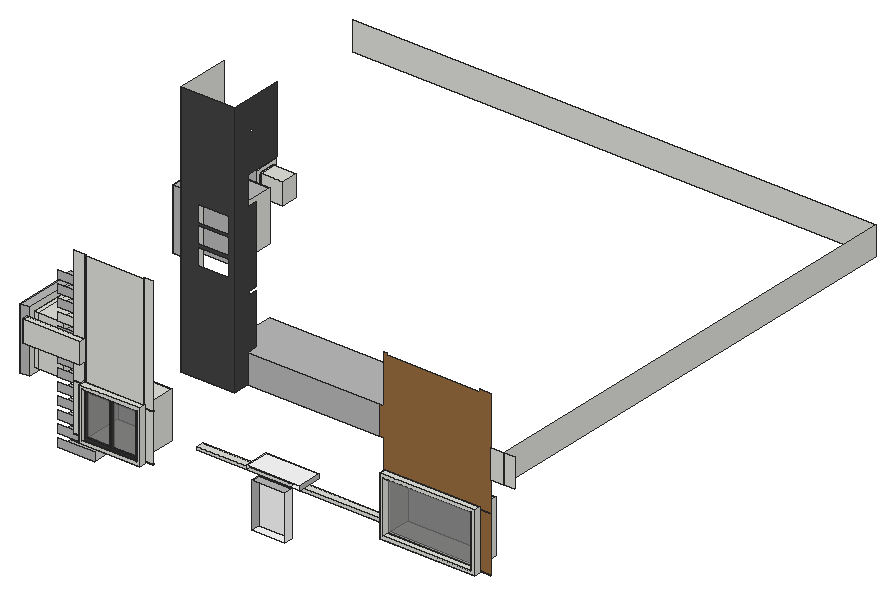
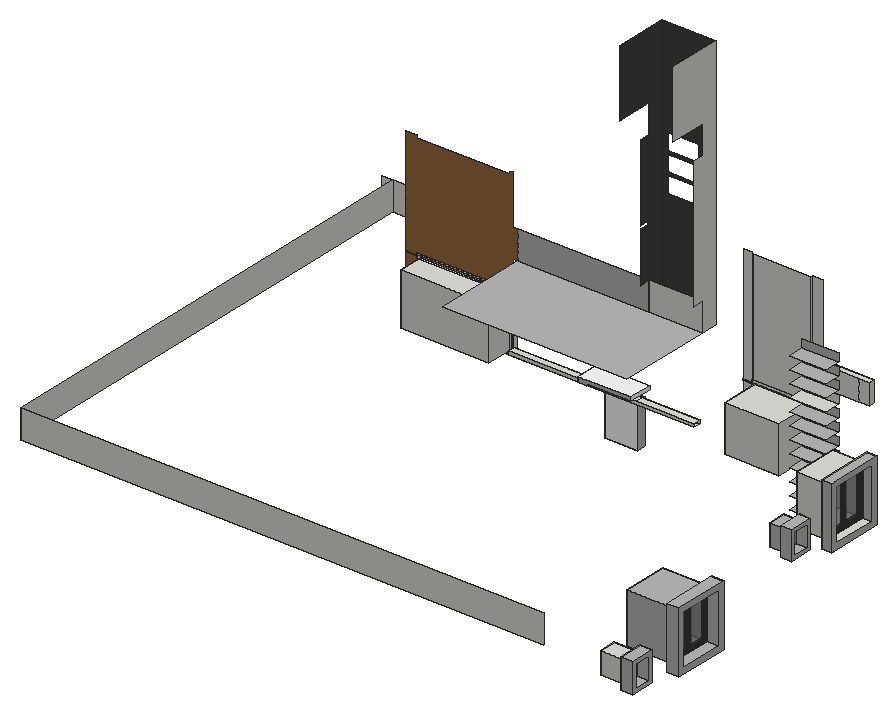
# SketchUp Ruby script. Lengths in inches.
U = 1.inch
M = Sketchup.active_model
def pt(a) = Geom::Point3d.new(a.map { |v| v * U })
def face(e, loops, mat)
  f = e.add_face(loops[0].map { |a| pt(a) })
  loops[1..].each { |l| e.add_face(l.map { |a| pt(a) }).erase! }
  f.material = f.back_material = mat if mat
  f
end
# faces: each face lists its corners as indices into pts; further lists are holes
def faces(e, pts, list, mat = nil) = list.each { |f| face(e, (f[0].is_a?(Array) ? f : [f]).map { |l| l.map { |i| pts[i] } }, mat) }
# xy, xz, yz: faces in a plane at the given z, y or x. An outline is a flat list of corners, or four numbers for a rectangle; further outlines are holes
def ring(l) = l.size == 4 ? [[l[0], l[1]], [l[2], l[1]], [l[2], l[3]], [l[0], l[3]]] : l.each_slice(2).to_a
def flat(e, list, mat, &to3) = list.each { |f| face(e, (f[0].is_a?(Array) ? f : [f]).map { |l| ring(l).map { |u, v| to3.(u, v) } }, mat) }
def xy(e, z, list, mat = nil) = flat(e, list, mat) { |x, y| [x, y, z] }
def xz(e, y, list, mat = nil) = flat(e, list, mat) { |x, z| [x, y, z] }
def yz(e, x, list, mat = nil) = flat(e, list, mat) { |y, z| [x, y, z] }
def lines(e, pts, list) = list.each { |a, b| e.add_line(pt(pts[a]), pt(pts[b])) }
# prism: a flat outline (further loops are holes) pulled along v
def prism(e, loops, v, mat = nil)
  f = face(e, loops, mat); d = Geom::Vector3d.new(v.map { |x| x * U })
  f.pushpull(f.normal.samedirection?(d) ? d.length : -d.length)
end
def box(e, o, s, mat = nil) = prism(e, [[o, [o[0] + s[0], o[1], o[2]], [o[0] + s[0], o[1] + s[1], o[2]], [o[0], o[1] + s[1], o[2]]]], [0, 0, s[2]], mat)
def at(x, y, z, deg = 0) = Geom::Transformation.translation(pt([x, y, z])) * Geom::Transformation.rotation(ORIGIN, Z_AXIS, deg.degrees)
def axes(o, x, y, z) = Geom::Transformation.new([*x, 0, *y, 0, *z, 0, *pt(o).to_a, 1])
def part(name) = M.definitions.add(name)
# library, detail: a bought-in or finely detailed component or shape, given as its bounding box
def library(name, o, s) = part(name).tap { |d| box(d.entities, o, s) }
def detail(e, o, s) = box(e.add_group.entities, o, s)
def put(e, d, t, mat = nil) = e.add_instance(d, t).tap { |i| i.material = mat if mat }
def group(e, t, mat = nil) = e.add_group.tap { |g| g.transformation = t; g.material = mat if mat }.entities
root = M.entities
M.materials.add("Generic").color = [155, 110, 63]
M.materials.add("Generic\#2").color = [186, 186, 186]
M.materials.add("[Color M00]").color = [255, 255, 255]
M.materials.add("[Color M07]").color = [58, 58, 58]
M.materials.add("[Granite Dark Gray]").color = [68, 67, 67]
M.materials.add("[Translucent Glass Gray]").color = [127, 127, 127]
M.materials["[Translucent Glass Gray]"].alpha = 0.58
M.materials.add("[Translucent Glass Gray]1").color = [127, 127, 127]
M.materials["[Translucent Glass Gray]1"].alpha = 0.5
c1 = part("Group\#1")
xy(c1.entities,0,[[0,0,46.77,20.375]])
xz(c1.entities,0,[[0,0,46.77,11.0625]])
c2 = part("Group\#3")
xy(c2.entities,0,[[0,0,70.4375,6]],"[Color M07]")
xy(c2.entities,2.83,[[2.83,0,33.8,3],[36.63,0,67.61,3]],"[Color M07]")
xy(c2.entities,56.73,[[2.83,0,33.8,3],[36.63,0,67.61,3]],"[Color M07]")
xy(c2.entities,59.5625,[[0,0,70.4375,6]],"[Color M07]")
xz(c2.entities,0,[[[0,0,70.4375,59.5625],[2.83,2.83,33.8,56.73],[36.63,2.83,67.61,56.73]]],"[Color M07]")
xz(c2.entities,3,[[2.83,2.83,33.8,56.73],[36.63,2.83,67.61,56.73]],"[Translucent Glass Gray]")
xz(c2.entities,6,[[0,0,70.4375,59.5625]],"[Translucent Glass Gray]")
yz(c2.entities,0,[[0,0,6,59.5625]],"[Color M07]")
yz(c2.entities,2.83,[[0,2.83,3,56.73]],"[Color M07]")
yz(c2.entities,33.8,[[0,2.83,3,56.73]],"[Color M07]")
yz(c2.entities,36.63,[[0,2.83,3,56.73]],"[Color M07]")
yz(c2.entities,67.61,[[0,2.83,3,56.73]],"[Color M07]")
yz(c2.entities,70.4375,[[0,0,6,59.5625]],"[Color M07]")
c3 = part("Group\#4")
xy(c3.entities,0,[[0,0,6,57.4375]],"[Color M07]")
xy(c3.entities,5.48,[[0,5.48,3,25.98],[0,31.46,3,51.96]],"[Color M07]")
xy(c3.entities,59.46,[[0,5.48,3,25.98],[0,31.46,3,51.96]],"[Color M07]")
xy(c3.entities,64.9375,[[0,0,6,57.4375]],"[Color M07]")
xz(c3.entities,0,[[0,0,6,64.9375]],"[Color M07]")
xz(c3.entities,5.48,[[0,5.48,3,59.46]],"[Color M07]")
xz(c3.entities,25.98,[[0,5.48,3,59.46]],"[Color M07]")
xz(c3.entities,31.46,[[0,5.48,3,59.46]],"[Color M07]")
xz(c3.entities,51.96,[[0,5.48,3,59.46]],"[Color M07]")
xz(c3.entities,57.4375,[[0,0,6,64.9375]],"[Color M07]")
yz(c3.entities,0,[[[0,0,57.4375,64.9375],[31.46,5.48,51.96,59.46],[5.48,5.48,25.98,59.46]]],"[Color M07]")
yz(c3.entities,3,[[5.48,5.48,25.98,59.46],[31.46,5.48,51.96,59.46]],"[Translucent Glass Gray]1")
yz(c3.entities,6,[[0,0,57.4375,64.9375]],"[Translucent Glass Gray]1")
c4 = part("Group\#2")
xy(c4.entities,0,[[0,0,113.875,3]])
xy(c4.entities,67.5625,[[0,0,113.875,3]])
xz(c4.entities,0,[[0,0,113.875,67.5625]],"[Translucent Glass Gray]")
xz(c4.entities,3,[[0,0,113.875,67.5625]],"[Translucent Glass Gray]")
yz(c4.entities,0,[[0,0,3,67.5625]])
yz(c4.entities,113.875,[[0,0,3,67.5625]])
c5 = part("Group\#5")
xy(c5.entities,0,[[0,0,3,21.5625]])
xy(c5.entities,28.3125,[[0,0,3,21.5625]])
xz(c5.entities,0,[[0,0,3,28.3125]])
xz(c5.entities,21.5625,[[0,0,3,28.3125]])
yz(c5.entities,0,[[0,0,21.5625,28.3125]],"[Translucent Glass Gray]1")
yz(c5.entities,3,[[0,0,21.5625,28.3125]],"[Translucent Glass Gray]1")
xy(root,621.53,[[370.16,118.5625,412.84,129.4375]],"[Color M00]")
xy(root,663.96,[[0,454.08,15.3125,525.8]],"Generic\#2")
xy(root,664.625,[[170.35,89.25,249.19,97.25],[171.66,97.25,172.16,98.375],[247.01,97.25,247.51,98.375]])
xy(root,666.77,[[36.4375,161.95,48.5,234.18]],"Generic\#2")
xy(root,667,[[157.47,97.25,170.35,98],[249.19,97.25,259.3125,98]])
xy(root,667.5,[[157.47,97.25,170.35,98],[249.19,97.25,259.3125,98]])
xy(root,668.33,[[174.55,89.25,244.99,97.25],[174.55,97.25,244.99,145.8125]])
xy(root,670.65,[[536.25,116.625,658.53,124.5]])
xy(root,671.1,[[0,461.22,72.5625,518.66]],"Generic\#2")
xy(root,674.16,[[36.4375,169.34,48.5,226.78],[48.5,169.34,87,226.78]])
xy(root,674.85,[[540.45,116.625,654.33,124.5],[540.45,124.5,654.33,156.8125]])
xy(root,675.92,[[0,569.11,15.3125,600.66]],"Generic\#2")
xy(root,678.86,[[370.16,118.5625,412.84,129.4375]],"Generic\#2")
xy(root,679.96,[[512.54,132.04,512.75,132.07,512.95,132.15,513.12,132.28,513.25,132.45,513.33,132.64,513.36,132.85,513.33,133.06,513.25,133.26,513.12,133.43,512.95,133.56,512.75,133.64,512.54,133.67,512.33,133.64,512.14,133.56,511.97,133.43,511.84,133.26,511.76,133.06,511.73,132.85,511.76,132.64,511.84,132.45,511.97,132.28,512.14,132.15,512.33,132.07],[518.54,132.04,518.75,132.07,518.95,132.15,519.12,132.28,519.25,132.45,519.33,132.64,519.36,132.85,519.33,133.06,519.25,133.26,519.12,133.43,518.95,133.56,518.75,133.64,518.54,133.67,518.33,133.64,518.14,133.56,517.97,133.43,517.84,133.26,517.76,133.06,517.73,132.85,517.76,132.64,517.84,132.45,517.97,132.28,518.14,132.15,518.33,132.07]])
xy(root,680.58,[[[290.4375,129.43,528.75,138.74],[506.67,132.04,506.88,132.07,507.07,132.15,507.24,132.28,507.37,132.45,507.45,132.64,507.48,132.85,507.45,133.06,507.37,133.26,507.24,133.43,507.07,133.56,506.88,133.64,506.67,133.67,506.46,133.64,506.26,133.56,506.09,133.43,505.96,133.26,505.88,133.06,505.86,132.85,505.88,132.64,505.96,132.45,506.09,132.28,506.26,132.15,506.46,132.07],[500.86,132.04,501.07,132.07,501.26,132.15,501.43,132.28,501.56,132.45,501.64,132.64,501.67,132.85,501.64,133.06,501.56,133.26,501.43,133.43,501.26,133.56,501.07,133.64,500.86,133.67,500.64,133.64,500.45,133.56,500.28,133.43,500.15,133.26,500.07,133.06,500.04,132.85,500.07,132.64,500.15,132.45,500.28,132.28,500.45,132.15,500.64,132.07],[494.92,132.04,495.13,132.07,495.32,132.15,495.49,132.28,495.62,132.45,495.7,132.64,495.73,132.85,495.7,133.06,495.62,133.26,495.49,133.43,495.32,133.56,495.13,133.64,494.92,133.67,494.71,133.64,494.51,133.56,494.34,133.43,494.21,133.26,494.13,133.06,494.11,132.85,494.13,132.64,494.21,132.45,494.34,132.28,494.51,132.15,494.71,132.07],[488.98,132.04,489.19,132.07,489.39,132.15,489.55,132.28,489.68,132.45,489.77,132.64,489.79,132.85,489.77,133.06,489.68,133.26,489.55,133.43,489.39,133.56,489.19,133.64,488.98,133.67,488.77,133.64,488.57,133.56,488.41,133.43,488.28,133.26,488.2,133.06,488.17,132.85,488.2,132.64,488.28,132.45,488.41,132.28,488.57,132.15,488.77,132.07],[483.11,132.04,483.32,132.07,483.51,132.15,483.68,132.28,483.81,132.45,483.89,132.64,483.92,132.85,483.89,133.06,483.81,133.26,483.68,133.43,483.51,133.56,483.32,133.64,483.11,133.67,482.89,133.64,482.7,133.56,482.53,133.43,482.4,133.26,482.32,133.06,482.29,132.85,482.32,132.64,482.4,132.45,482.53,132.28,482.7,132.15,482.89,132.07],[477.23,132.04,477.44,132.07,477.64,132.15,477.8,132.28,477.93,132.45,478.02,132.64,478.04,132.85,478.02,133.06,477.93,133.26,477.8,133.43,477.64,133.56,477.44,133.64,477.23,133.67,477.02,133.64,476.82,133.56,476.66,133.43,476.53,133.26,476.45,133.06,476.42,132.85,476.45,132.64,476.53,132.45,476.66,132.28,476.82,132.15,477.02,132.07],[471.54,132.04,471.75,132.07,471.95,132.15,472.12,132.28,472.25,132.45,472.33,132.64,472.36,132.85,472.33,133.06,472.25,133.26,472.12,133.43,471.95,133.56,471.75,133.64,471.54,133.67,471.33,133.64,471.14,133.56,470.97,133.43,470.84,133.26,470.76,133.06,470.73,132.85,470.76,132.64,470.84,132.45,470.97,132.28,471.14,132.15,471.33,132.07],[465.54,132.04,465.75,132.07,465.95,132.15,466.12,132.28,466.25,132.45,466.33,132.64,466.36,132.85,466.33,133.06,466.25,133.26,466.12,133.43,465.95,133.56,465.75,133.64,465.54,133.67,465.33,133.64,465.14,133.56,464.97,133.43,464.84,133.26,464.76,133.06,464.73,132.85,464.76,132.64,464.84,132.45,464.97,132.28,465.14,132.15,465.33,132.07],[459.48,132.04,459.69,132.07,459.89,132.15,460.05,132.28,460.18,132.45,460.27,132.64,460.29,132.85,460.27,133.06,460.18,133.26,460.05,133.43,459.89,133.56,459.69,133.64,459.48,133.67,459.27,133.64,459.07,133.56,458.91,133.43,458.78,133.26,458.7,133.06,458.67,132.85,458.7,132.64,458.78,132.45,458.91,132.28,459.07,132.15,459.27,132.07],[453.86,132.04,454.07,132.07,454.26,132.15,454.43,132.28,454.56,132.45,454.64,132.64,454.67,132.85,454.64,133.06,454.56,133.26,454.43,133.43,454.26,133.56,454.07,133.64,453.86,133.67,453.64,133.64,453.45,133.56,453.28,133.43,453.15,133.26,453.07,133.06,453.04,132.85,453.07,132.64,453.15,132.45,453.28,132.28,453.45,132.15,453.64,132.07],[447.98,132.04,448.19,132.07,448.39,132.15,448.55,132.28,448.68,132.45,448.77,132.64,448.79,132.85,448.77,133.06,448.68,133.26,448.55,133.43,448.39,133.56,448.19,133.64,447.98,133.67,447.77,133.64,447.57,133.56,447.41,133.43,447.28,133.26,447.2,133.06,447.17,132.85,447.2,132.64,447.28,132.45,447.41,132.28,447.57,132.15,447.77,132.07],[442.11,132.04,442.32,132.07,442.51,132.15,442.68,132.28,442.81,132.45,442.89,132.64,442.92,132.85,442.89,133.06,442.81,133.26,442.68,133.43,442.51,133.56,442.32,133.64,442.11,133.67,441.89,133.64,441.7,133.56,441.53,133.43,441.4,133.26,441.32,133.06,441.29,132.85,441.32,132.64,441.4,132.45,441.53,132.28,441.7,132.15,441.89,132.07],[436.11,132.04,436.32,132.07,436.51,132.15,436.68,132.28,436.81,132.45,436.89,132.64,436.92,132.85,436.89,133.06,436.81,133.26,436.68,133.43,436.51,133.56,436.32,133.64,436.11,133.67,435.89,133.64,435.7,133.56,435.53,133.43,435.4,133.26,435.32,133.06,435.29,132.85,435.32,132.64,435.4,132.45,435.53,132.28,435.7,132.15,435.89,132.07],[430.54,132.04,430.75,132.07,430.95,132.15,431.12,132.28,431.25,132.45,431.33,132.64,431.36,132.85,431.33,133.06,431.25,133.26,431.12,133.43,430.95,133.56,430.75,133.64,430.54,133.67,430.33,133.64,430.14,133.56,429.97,133.43,429.84,133.26,429.76,133.06,429.73,132.85,429.76,132.64,429.84,132.45,429.97,132.28,430.14,132.15,430.33,132.07],[424.36,132.04,424.57,132.07,424.76,132.15,424.93,132.28,425.06,132.45,425.14,132.64,425.17,132.85,425.14,133.06,425.06,133.26,424.93,133.43,424.76,133.56,424.57,133.64,424.36,133.67,424.14,133.64,423.95,133.56,423.78,133.43,423.65,133.26,423.57,133.06,423.54,132.85,423.57,132.64,423.65,132.45,423.78,132.28,423.95,132.15,424.14,132.07],[418.54,132.04,418.75,132.07,418.95,132.15,419.12,132.28,419.25,132.45,419.33,132.64,419.36,132.85,419.33,133.06,419.25,133.26,419.12,133.43,418.95,133.56,418.75,133.64,418.54,133.67,418.33,133.64,418.14,133.56,417.97,133.43,417.84,133.26,417.76,133.06,417.73,132.85,417.76,132.64,417.84,132.45,417.97,132.28,418.14,132.15,418.33,132.07],[412.67,132.04,412.88,132.07,413.07,132.15,413.24,132.28,413.37,132.45,413.45,132.64,413.48,132.85,413.45,133.06,413.37,133.26,413.24,133.43,413.07,133.56,412.88,133.64,412.67,133.67,412.46,133.64,412.26,133.56,412.09,133.43,411.96,133.26,411.88,133.06,411.86,132.85,411.88,132.64,411.96,132.45,412.09,132.28,412.26,132.15,412.46,132.07],[406.79,132.04,407,132.07,407.2,132.15,407.37,132.28,407.5,132.45,407.58,132.64,407.61,132.85,407.58,133.06,407.5,133.26,407.37,133.43,407.2,133.56,407,133.64,406.79,133.67,406.58,133.64,406.39,133.56,406.22,133.43,406.09,133.26,406.01,133.06,405.98,132.85,406.01,132.64,406.09,132.45,406.22,132.28,406.39,132.15,406.58,132.07],[400.92,132.04,401.13,132.07,401.32,132.15,401.49,132.28,401.62,132.45,401.7,132.64,401.73,132.85,401.7,133.06,401.62,133.26,401.49,133.43,401.32,133.56,401.13,133.64,400.92,133.67,400.71,133.64,400.51,133.56,400.34,133.43,400.21,133.26,400.13,133.06,400.11,132.85,400.13,132.64,400.21,132.45,400.34,132.28,400.51,132.15,400.71,132.07],[394.86,132.04,395.07,132.07,395.26,132.15,395.43,132.28,395.56,132.45,395.64,132.64,395.67,132.85,395.64,133.06,395.56,133.26,395.43,133.43,395.26,133.56,395.07,133.64,394.86,133.67,394.64,133.64,394.45,133.56,394.28,133.43,394.15,133.26,394.07,133.06,394.04,132.85,394.07,132.64,394.15,132.45,394.28,132.28,394.45,132.15,394.64,132.07],[389.17,132.04,389.38,132.07,389.57,132.15,389.74,132.28,389.87,132.45,389.95,132.64,389.98,132.85,389.95,133.06,389.87,133.26,389.74,133.43,389.57,133.56,389.38,133.64,389.17,133.67,388.96,133.64,388.76,133.56,388.59,133.43,388.46,133.26,388.38,133.06,388.36,132.85,388.38,132.64,388.46,132.45,388.59,132.28,388.76,132.15,388.96,132.07],[383.23,132.04,383.44,132.07,383.64,132.15,383.8,132.28,383.93,132.45,384.02,132.64,384.04,132.85,384.02,133.06,383.93,133.26,383.8,133.43,383.64,133.56,383.44,133.64,383.23,133.67,383.02,133.64,382.82,133.56,382.66,133.43,382.53,133.26,382.45,133.06,382.42,132.85,382.45,132.64,382.53,132.45,382.66,132.28,382.82,132.15,383.02,132.07],[377.42,132.04,377.63,132.07,377.82,132.15,377.99,132.28,378.12,132.45,378.2,132.64,378.23,132.85,378.2,133.06,378.12,133.26,377.99,133.43,377.82,133.56,377.63,133.64,377.42,133.67,377.21,133.64,377.01,133.56,376.84,133.43,376.71,133.26,376.63,133.06,376.61,132.85,376.63,132.64,376.71,132.45,376.84,132.28,377.01,132.15,377.21,132.07],[371.48,132.04,371.69,132.07,371.89,132.15,372.05,132.28,372.18,132.45,372.27,132.64,372.29,132.85,372.27,133.06,372.18,133.26,372.05,133.43,371.89,133.56,371.69,133.64,371.48,133.67,371.27,133.64,371.07,133.56,370.91,133.43,370.78,133.26,370.7,133.06,370.67,132.85,370.7,132.64,370.78,132.45,370.91,132.28,371.07,132.15,371.27,132.07],[365.67,132.04,365.88,132.07,366.07,132.15,366.24,132.28,366.37,132.45,366.45,132.64,366.48,132.85,366.45,133.06,366.37,133.26,366.24,133.43,366.07,133.56,365.88,133.64,365.67,133.67,365.46,133.64,365.26,133.56,365.09,133.43,364.96,133.26,364.88,133.06,364.86,132.85,364.88,132.64,364.96,132.45,365.09,132.28,365.26,132.15,365.46,132.07],[359.86,132.04,360.07,132.07,360.26,132.15,360.43,132.28,360.56,132.45,360.64,132.64,360.67,132.85,360.64,133.06,360.56,133.26,360.43,133.43,360.26,133.56,360.07,133.64,359.86,133.67,359.64,133.64,359.45,133.56,359.28,133.43,359.15,133.26,359.07,133.06,359.04,132.85,359.07,132.64,359.15,132.45,359.28,132.28,359.45,132.15,359.64,132.07],[353.79,132.04,354,132.07,354.2,132.15,354.37,132.28,354.5,132.45,354.58,132.64,354.61,132.85,354.58,133.06,354.5,133.26,354.37,133.43,354.2,133.56,354,133.64,353.79,133.67,353.58,133.64,353.39,133.56,353.22,133.43,353.09,133.26,353.01,133.06,352.98,132.85,353.01,132.64,353.09,132.45,353.22,132.28,353.39,132.15,353.58,132.07],[348.23,132.04,348.44,132.07,348.64,132.15,348.8,132.28,348.93,132.45,349.02,132.64,349.04,132.85,349.02,133.06,348.93,133.26,348.8,133.43,348.64,133.56,348.44,133.64,348.23,133.67,348.02,133.64,347.82,133.56,347.66,133.43,347.53,133.26,347.45,133.06,347.42,132.85,347.45,132.64,347.53,132.45,347.66,132.28,347.82,132.15,348.02,132.07],[342.23,132.04,342.44,132.07,342.64,132.15,342.8,132.28,342.93,132.45,343.02,132.64,343.04,132.85,343.02,133.06,342.93,133.26,342.8,133.43,342.64,133.56,342.44,133.64,342.23,133.67,342.02,133.64,341.82,133.56,341.66,133.43,341.53,133.26,341.45,133.06,341.42,132.85,341.45,132.64,341.53,132.45,341.66,132.28,341.82,132.15,342.02,132.07],[336.36,132.04,336.57,132.07,336.76,132.15,336.93,132.28,337.06,132.45,337.14,132.64,337.17,132.85,337.14,133.06,337.06,133.26,336.93,133.43,336.76,133.56,336.57,133.64,336.36,133.67,336.14,133.64,335.95,133.56,335.78,133.43,335.65,133.26,335.57,133.06,335.54,132.85,335.57,132.64,335.65,132.45,335.78,132.28,335.95,132.15,336.14,132.07],[330.48,132.01,330.69,132.04,330.89,132.125,331.06,132.25,331.1875,132.42,331.27,132.62,331.3,132.83,331.27,133.04,331.1875,133.23,331.06,133.4,330.89,133.53,330.69,133.61,330.48,133.64,330.27,133.61,330.08,133.53,329.91,133.4,329.78,133.23,329.7,133.04,329.67,132.83,329.7,132.62,329.78,132.42,329.91,132.25,330.08,132.125,330.27,132.04],[324.98,132.01,325.19,132.04,325.39,132.125,325.56,132.25,325.6875,132.42,325.77,132.62,325.8,132.83,325.77,133.04,325.6875,133.23,325.56,133.4,325.39,133.53,325.19,133.61,324.98,133.64,324.77,133.61,324.58,133.53,324.41,133.4,324.28,133.23,324.2,133.04,324.17,132.83,324.2,132.62,324.28,132.42,324.41,132.25,324.58,132.125,324.77,132.04],[318.73,132.01,318.94,132.04,319.14,132.125,319.31,132.25,319.4375,132.42,319.52,132.62,319.55,132.83,319.52,133.04,319.4375,133.23,319.31,133.4,319.14,133.53,318.94,133.61,318.73,133.64,318.52,133.61,318.33,133.53,318.16,133.4,318.03,133.23,317.95,133.04,317.92,132.83,317.95,132.62,318.03,132.42,318.16,132.25,318.33,132.125,318.52,132.04],[312.8,132.01,313.01,132.04,313.2,132.125,313.37,132.25,313.5,132.42,313.58,132.62,313.61,132.83,313.58,133.04,313.5,133.23,313.37,133.4,313.2,133.53,313.01,133.61,312.8,133.64,312.58,133.61,312.39,133.53,312.22,133.4,312.09,133.23,312.01,133.04,311.98,132.83,312.01,132.62,312.09,132.42,312.22,132.25,312.39,132.125,312.58,132.04],[306.92,132.01,307.13,132.04,307.33,132.125,307.49,132.25,307.625,132.42,307.7,132.62,307.73,132.83,307.7,133.04,307.625,133.23,307.49,133.4,307.33,133.53,307.13,133.61,306.92,133.64,306.71,133.61,306.51,133.53,306.35,133.4,306.22,133.23,306.14,133.04,306.11,132.83,306.14,132.62,306.22,132.42,306.35,132.25,306.51,132.125,306.71,132.04],[294.98,132.01,295.19,132.04,295.39,132.125,295.56,132.25,295.6875,132.42,295.77,132.62,295.8,132.83,295.77,133.04,295.6875,133.23,295.56,133.4,295.39,133.53,295.19,133.61,294.98,133.64,294.77,133.61,294.58,133.53,294.41,133.4,294.28,133.23,294.2,133.04,294.17,132.83,294.2,132.62,294.28,132.42,294.41,132.25,294.58,132.125,294.77,132.04],[300.98,132.01,301.19,132.04,301.39,132.125,301.56,132.25,301.6875,132.42,301.77,132.62,301.8,132.83,301.77,133.04,301.6875,133.23,301.56,133.4,301.39,133.53,301.19,133.61,300.98,133.64,300.77,133.61,300.58,133.53,300.41,133.4,300.28,133.23,300.2,133.04,300.17,132.83,300.2,132.62,300.28,132.42,300.41,132.25,300.58,132.125,300.77,132.04]]])
xy(root,681.07,[[15.3125,574.26,44.75,595.82]])
xy(root,681.07,[[0,574.26,15.3125,595.82]],"Generic\#2")
xy(root,684.77,[[290.4375,129.43,363.4375,138.74],[363.4375,129.43,419.5625,138.74],[419.5625,129.43,528.75,138.74]])
xy(root,686.17,[[34.5,270.92,48.5,300.91]],"Generic\#2")
xy(root,687.77,[[419.5625,118.5625,431.875,149.5]],"[Color M00]")
xy(root,690.39,[[34.5,275.13,65.625,296.69]],"Generic\#2")
xy(root,694.14,[[363.4375,118.5625,431.875,149.5]],"[Color M00]")
xy(root,709.39,[[15.3125,574.26,44.75,595.82]])
xy(root,709.39,[[0,574.26,15.3125,595.82]],"Generic\#2")
xy(root,714.22,[[0,569.11,15.3125,600.66]],"Generic\#2")
xy(root,718.7,[[34.5,275.13,65.625,296.69]],"Generic\#2")
xy(root,722.91,[[34.5,270.92,48.5,300.91]],"Generic\#2")
xy(root,727.89,[[174.55,89.25,244.99,97.25],[174.55,97.25,244.99,145.8125]])
xy(root,728.25,[[157.47,97.25,170.35,98],[249.19,97.25,259.3125,98]])
xy(root,728.75,[[157.47,97.25,170.35,98],[249.19,97.25,259.3125,98]])
xy(root,732.09,[[170.35,89.25,249.19,97.25],[171.66,97.25,172.16,98],[247.01,97.25,247.51,98]])
xy(root,736.04,[[0,461.22,72.5625,518.66]],"Generic\#2")
xy(root,739.1,[[48.5,169.34,87,226.78]])
xy(root,739.1,[[36.4375,169.34,48.5,226.78]],"Generic\#2")
xy(root,742.41,[[540.45,116.625,654.33,124.5],[540.45,124.5,654.33,156.8125]])
xy(root,743.18,[[0,454.08,15.3125,525.8]],"Generic\#2")
xy(root,746.5,[[36.4375,161.95,48.5,234.18]],"Generic\#2")
xy(root,746.61,[[536.25,116.625,658.53,124.5]])
xy(root,754.57,[[96.98,89.5625,171.66,97.25]])
xy(root,781.48,[[96.98,89.5625,171.66,97.25]])
xy(root,782.8125,[[290.4375,124.5,528.75,246]],"Generic\#2")
xy(root,782.8125,[[290.4375,103.5,359.25,124.5]],"[Granite Dark Gray]")
xz(root,89.25,[[[170.35,664.625,249.19,732.09],[174.55,668.33,244.99,727.89]]])
xz(root,89.5625,[[96.98,754.57,171.66,781.48]])
xz(root,97.25,[[170.35,664.625,171.66,667],[171.66,664.625,247.01,667],[247.01,664.625,249.19,667],[170.35,667,171.66,728.75],[[171.66,667,247.01,728.75],[174.55,668.33,244.99,727.89]],
  [247.01,667,249.19,728.75],[157.47,667.5,170.35,728.25],[249.19,667.5,259.3125,728.25],[157.47,728.75,170.35,728.75,170.35,732.09,171.66,732.09,171.66,754.57,157.47,754.57],[170.35,728.75,171.66,732.09],
  [171.66,728.75,247.01,732.09],[247.01,728.75,249.19,732.09],[249.19,728.75,259.3125,728.75,259.3125,879.5,249.19,879.5,249.19,877.875,247.51,877.875,247.51,732.09,249.19,732.09],[172.16,732.09,247.01,877.875],[96.98,754.57,110.7,781.48],
  [110.7,754.57,157.47,781.48],[157.47,754.57,171.66,781.48],[157.47,781.48,171.66,781.48,171.66,877.875,170.35,877.875,170.35,879.5,157.47,879.5]])
xz(root,98,[[157.47,667,170.35,667.5],[249.19,667,259.3125,667.5],[157.47,728.25,170.35,728.75],[249.19,728.25,259.3125,728.75],[171.66,732.09,172.16,877.875],
  [247.01,732.09,247.51,877.875]])
xz(root,103.5,[[[290.4375,782.8125,359.25,1111.375],[312.22,912.72,352.19,934.81],[312.34,962.59,352.07,984.44],[312.34,937.71,352.07,959.57]]],"[Granite Dark Gray]")
xz(root,116.625,[[[536.25,670.65,658.53,746.61],[540.45,674.85,654.33,742.41]]])
xz(root,124.5,[[536.25,670.65,658.53,672.25],[[536.25,672.25,658.53,743.8125],[540.45,674.85,654.33,742.41]],[536.25,743.8125,658.53,746.61],[290.4375,782.8125,359.25,819.75],[673.48,782.8125,690.4375,819.75],
  [690.4375,782.8125,703.6875,819.75]])
xz(root,124.5,[[535.75,672.25,536.25,743.8125],[658.53,672.25,673.48,672.75],[658.53,672.75,673.48,743.3125],[658.53,743.3125,673.48,743.8125],[535.75,743.8125,536.25,743.8125,536.25,746.61,658.53,746.61,658.53,743.8125,673.48,743.8125,673.48,882.5,658.46,882.5,658.46,879.52,538.69,879.52,538.69,882.5,535.75,882.5,535.75,819.75,528.75,819.75,528.75,782.8125,535.75,782.8125]],"Generic")
xz(root,124.5,[[359.25,782.8125,528.75,819.75]],"Generic\#2")
xz(root,129.43,[[290.4375,680.58,528.75,684.77]])
xz(root,129.4375,[[370.16,621.53,412.84,678.86]],"[Color M00]")
xz(root,138.74,[[290.4375,680.58,528.75,684.77]])
xz(root,145.8125,[[174.55,668.33,244.99,727.89]])
xz(root,149.5,[[419.5625,687.77,419.5625,689.33,363.4375,689.33,363.4375,694.14,431.875,694.14,431.875,687.77]],"Generic\#2")
xz(root,156.8125,[[540.45,674.85,654.33,742.41]])
xz(root,161.95,[[36.4375,666.77,48.5,746.5]],"Generic\#2")
xz(root,169.34,[[48.5,674.16,87,739.1]])
xz(root,169.34,[[36.4375,674.16,48.5,739.1]],"Generic\#2")
xz(root,226.78,[[48.5,674.16,87,739.1]])
xz(root,226.78,[[36.4375,674.16,48.5,739.1]],"Generic\#2")
xz(root,234.18,[[36.4375,666.77,48.5,746.5]],"Generic\#2")
xz(root,270.92,[[34.5,686.17,48.5,722.91]],"Generic\#2")
xz(root,275.13,[[34.5,690.39,65.625,718.7]],"Generic\#2")
xz(root,296.69,[[34.5,690.39,65.625,718.7]],"Generic\#2")
xz(root,300.91,[[34.5,686.17,48.5,722.91]],"Generic\#2")
xz(root,454.08,[[0,663.96,15.3125,743.18]],"Generic\#2")
xz(root,461.22,[[0,671.1,72.5625,736.04]],"Generic\#2")
xz(root,518.66,[[0,671.1,72.5625,736.04]],"Generic\#2")
xz(root,525.8,[[0,663.96,15.3125,743.18]],"Generic\#2")
xz(root,569.11,[[0,675.92,15.3125,714.22]],"Generic\#2")
xz(root,574.26,[[15.3125,681.07,44.75,709.39]])
xz(root,574.26,[[0,681.07,15.3125,709.39]],"Generic\#2")
xz(root,595.82,[[15.3125,681.07,44.75,709.39]])
xz(root,595.82,[[0,681.07,15.3125,709.39]],"Generic\#2")
xz(root,600.66,[[0,675.92,15.3125,714.22]],"Generic\#2")
xz(root,724.5,[[15.3125,782.8125,690.4375,819.75]])
yz(root,0,[[[454.08,663.96,525.8,743.18],[461.22,671.1,518.66,736.04]],[[569.11,675.92,600.66,714.22],[574.26,681.07,595.82,709.39]]],"Generic\#2")
yz(root,15.3125,[[[569.11,675.92,600.66,714.22],[574.26,681.07,595.82,709.39]]])
yz(root,34.5,[[[270.92,686.17,300.91,722.91],[275.13,690.39,296.69,718.7]]],"Generic\#2")
yz(root,36.4375,[[[161.95,666.77,234.18,746.5],[169.34,674.16,226.78,739.1]]],"Generic\#2")
yz(root,44.75,[[574.26,681.07,595.82,709.39]])
yz(root,48.5,[[[161.95,666.77,234.18,746.5],[169.34,674.16,226.78,739.1]]])
yz(root,65.625,[[275.13,690.39,296.69,718.7]])
yz(root,72.5625,[[461.22,671.1,518.66,736.04]])
yz(root,87,[[169.34,674.16,226.78,739.1]])
yz(root,96.98,[[89.5625,754.57,97.25,781.48]])
yz(root,170.35,[[89.25,664.625,97.25,732.09],[97.25,667,98,667.5],[97.25,728.25,98,728.75]])
yz(root,171.66,[[97.25,732.09,98,754.57],[89.5625,754.57,97.25,781.48],[97.25,754.57,98,781.48],[97.25,781.48,98,877.875]])
yz(root,172.16,[[97.25,732.09,98,754.57],[97.25,754.57,98,781.48],[97.25,781.48,98,877.875]])
yz(root,174.55,[[89.25,668.33,97.25,727.89],[97.25,668.33,145.8125,727.89]])
yz(root,244.99,[[89.25,668.33,97.25,727.89],[97.25,668.33,145.8125,727.89]])
yz(root,247.01,[[97.25,732.09,98,754.57],[97.25,754.57,98,781.48],[97.25,781.48,98,877.875]])
yz(root,247.51,[[97.25,732.09,98,754.57],[97.25,754.57,98,781.48],[97.25,781.48,98,877.875]])
yz(root,249.19,[[89.25,664.625,97.25,732.09],[97.25,667,98,667.5],[97.25,728.25,98,728.75]])
yz(root,290.4375,[[103.5,782.8125,124.5,782.8125,124.5,819.75,138.74,819.75,138.74,987.75,124.5,987.75,124.5,1024.6875,172.5,1024.6875,172.5,1111.375,103.5,1111.375]])
yz(root,359.25,[[[103.5,782.8125,124.5,782.8125,124.5,819.75,138.74,819.75,138.74,884.89,127.31,884.89,127.31,889.08,138.74,889.08,138.74,987.75,124.5,987.75,124.5,1024.6875,172.5,1024.6875,172.5,1111.375,103.5,1111.375],[128.48,1072.38,133.48,1075.32]]],"[Granite Dark Gray]")
yz(root,363.4375,[[118.5625,689.33,149.5,694.14]],"[Color M00]")
yz(root,370.16,[[118.5625,621.53,129.4375,678.86]],"Generic\#2")
yz(root,412.84,[[118.5625,621.53,129.4375,678.86]],"[Color M00]")
yz(root,431.875,[[118.5625,687.77,149.5,694.14]],"Generic\#2")
yz(root,536.25,[[116.625,670.65,124.5,746.61]])
yz(root,540.45,[[116.625,674.85,124.5,742.41],[124.5,674.85,156.8125,742.41]])
yz(root,654.33,[[116.625,674.85,124.5,742.41],[124.5,674.85,156.8125,742.41]])
yz(root,658.53,[[116.625,670.65,124.5,746.61]])
yz(root,690.4375,[[124.5,782.8125,724.5,819.75]])
p = [[528.75,134.28,682.46],[290.4375,134.28,682.46]]
lines(root,p,[[0,1]])
put(root,c1,at(110.7,130.3125,620.5625),"Generic\#2")
put(root,c1,at(110.7,130.3125,636.75),"Generic\#2")
put(root,c1,at(110.7,130.3125,652.9375),"Generic\#2")
put(root,c2,at(174.55,91.75,668.33))
put(root,c1,at(110.7,130.3125,669.125),"Generic\#2")
put(root,c3,at(15.3125,461.22,671.1))
put(root,c3,at(48.5,169.34,674.16))
put(root,c4,at(540.45,124.5,674.85))
put(root,c5,at(15.3125,574.26,681.07))
put(root,c1,at(110.7,130.3125,685.3125),"Generic\#2")
put(root,c5,at(48.5,275.13,690.39))
put(root,c1,at(110.7,130.3125,701.5),"Generic\#2")
put(root,c1,at(110.7,130.3125,717.6875),"Generic\#2")
put(root,c1,at(110.7,130.3125,733.875),"Generic\#2")
put(root,c1,at(110.7,130.3125,750.0625),"Generic\#2")
put(root,c1,at(110.7,130.3125,766.25))
put(root,c1,at(110.7,130.3125,782.4375),"Generic\#2")
put(root,c1,at(110.7,130.3125,798.625),"Generic\#2")
put(root,c1,at(110.7,130.3125,814.8125),"Generic\#2")
